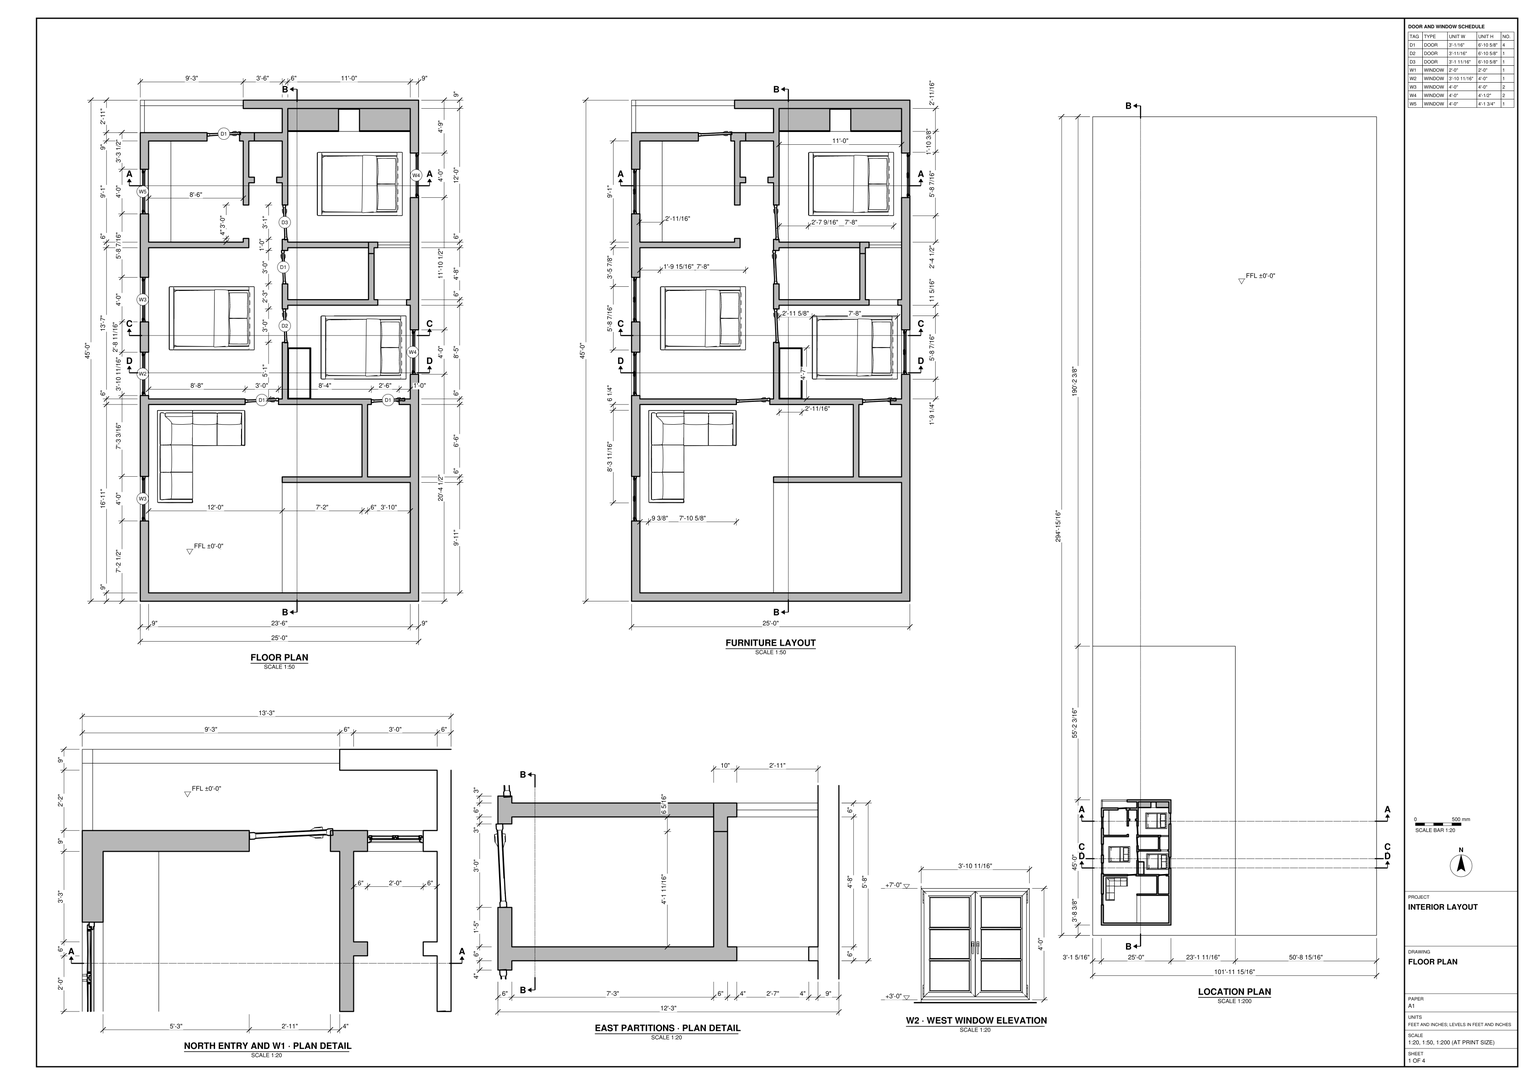
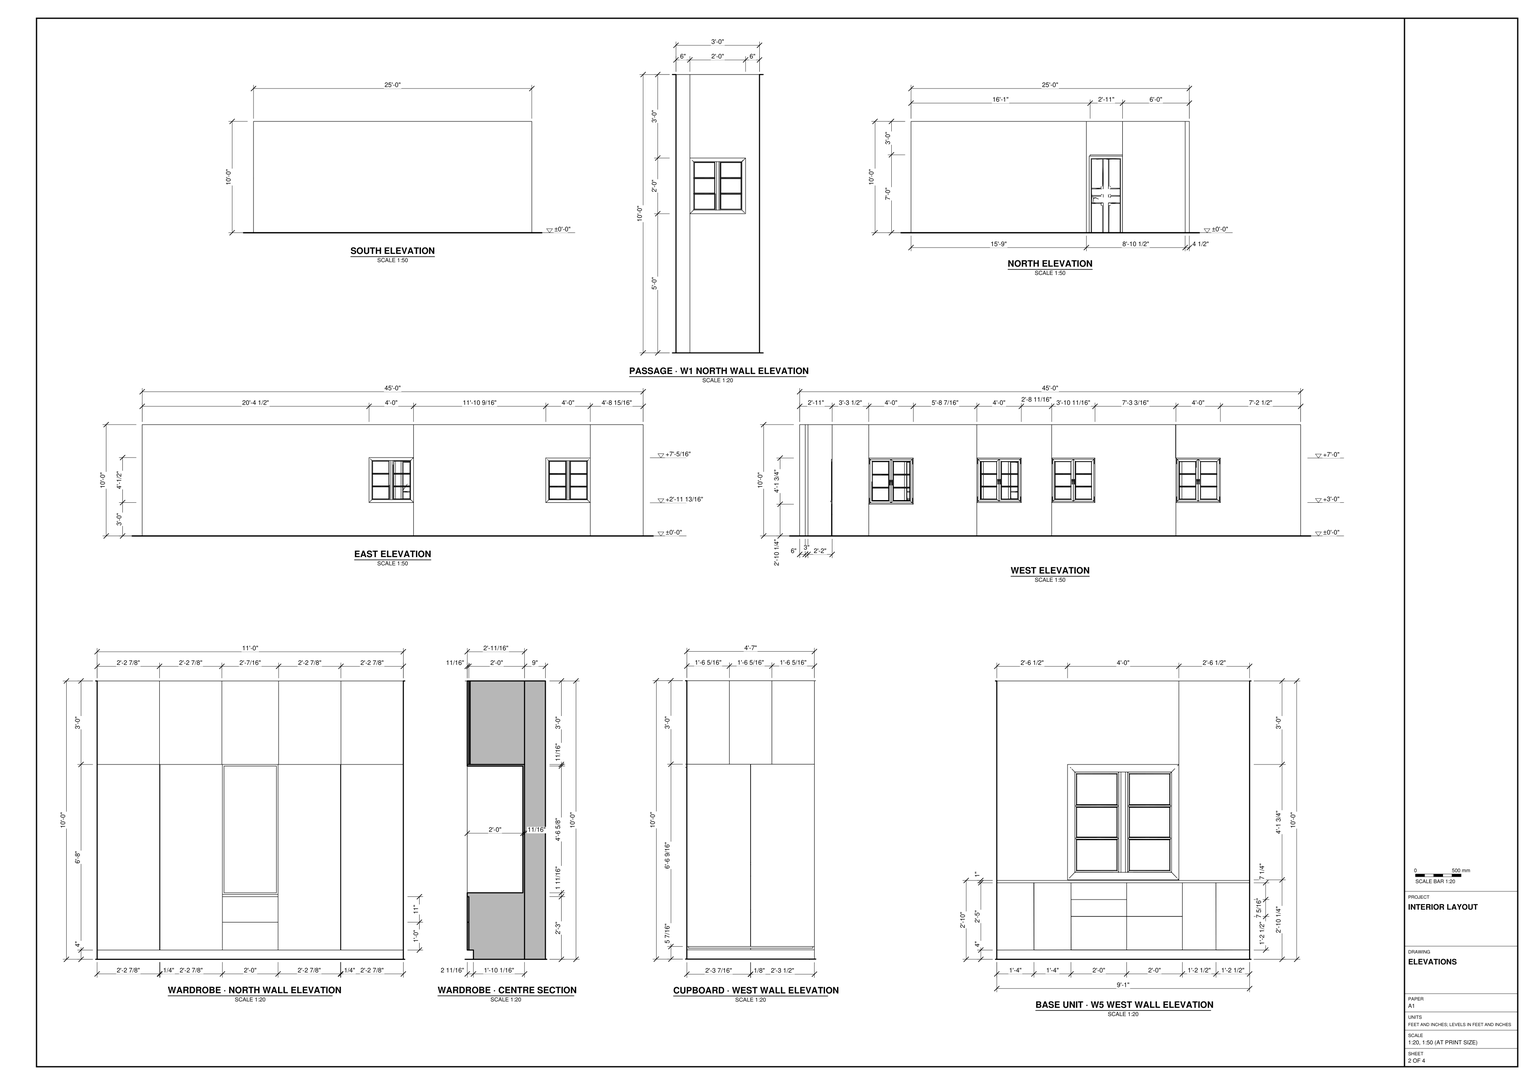
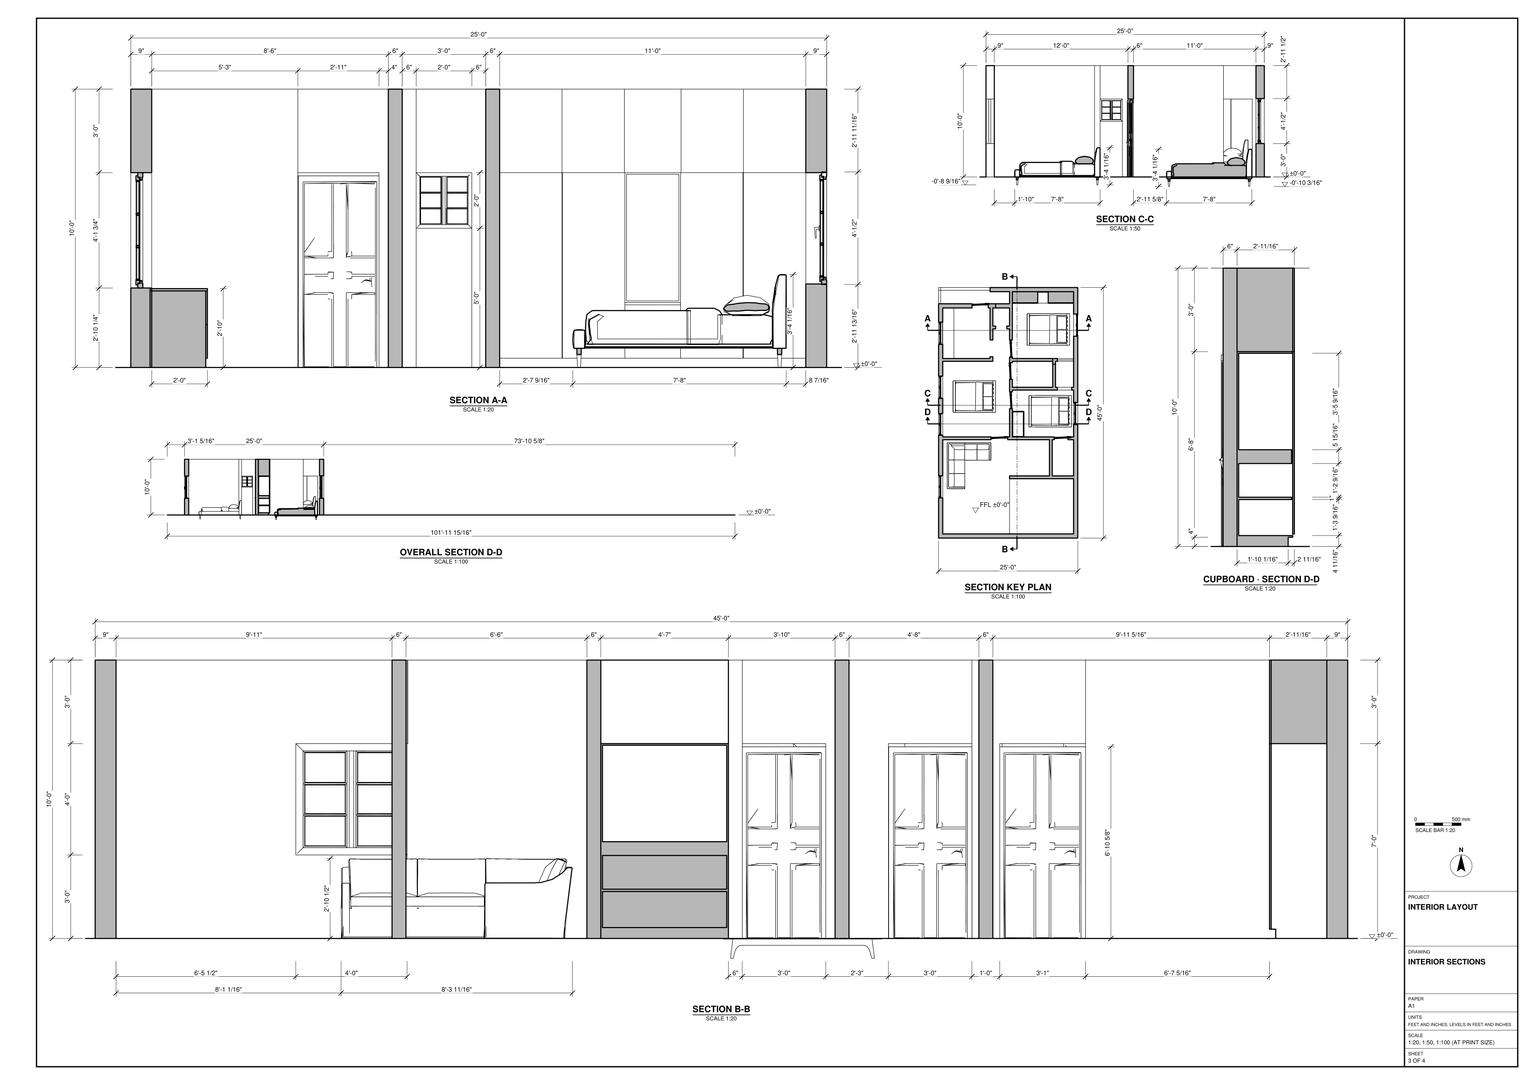
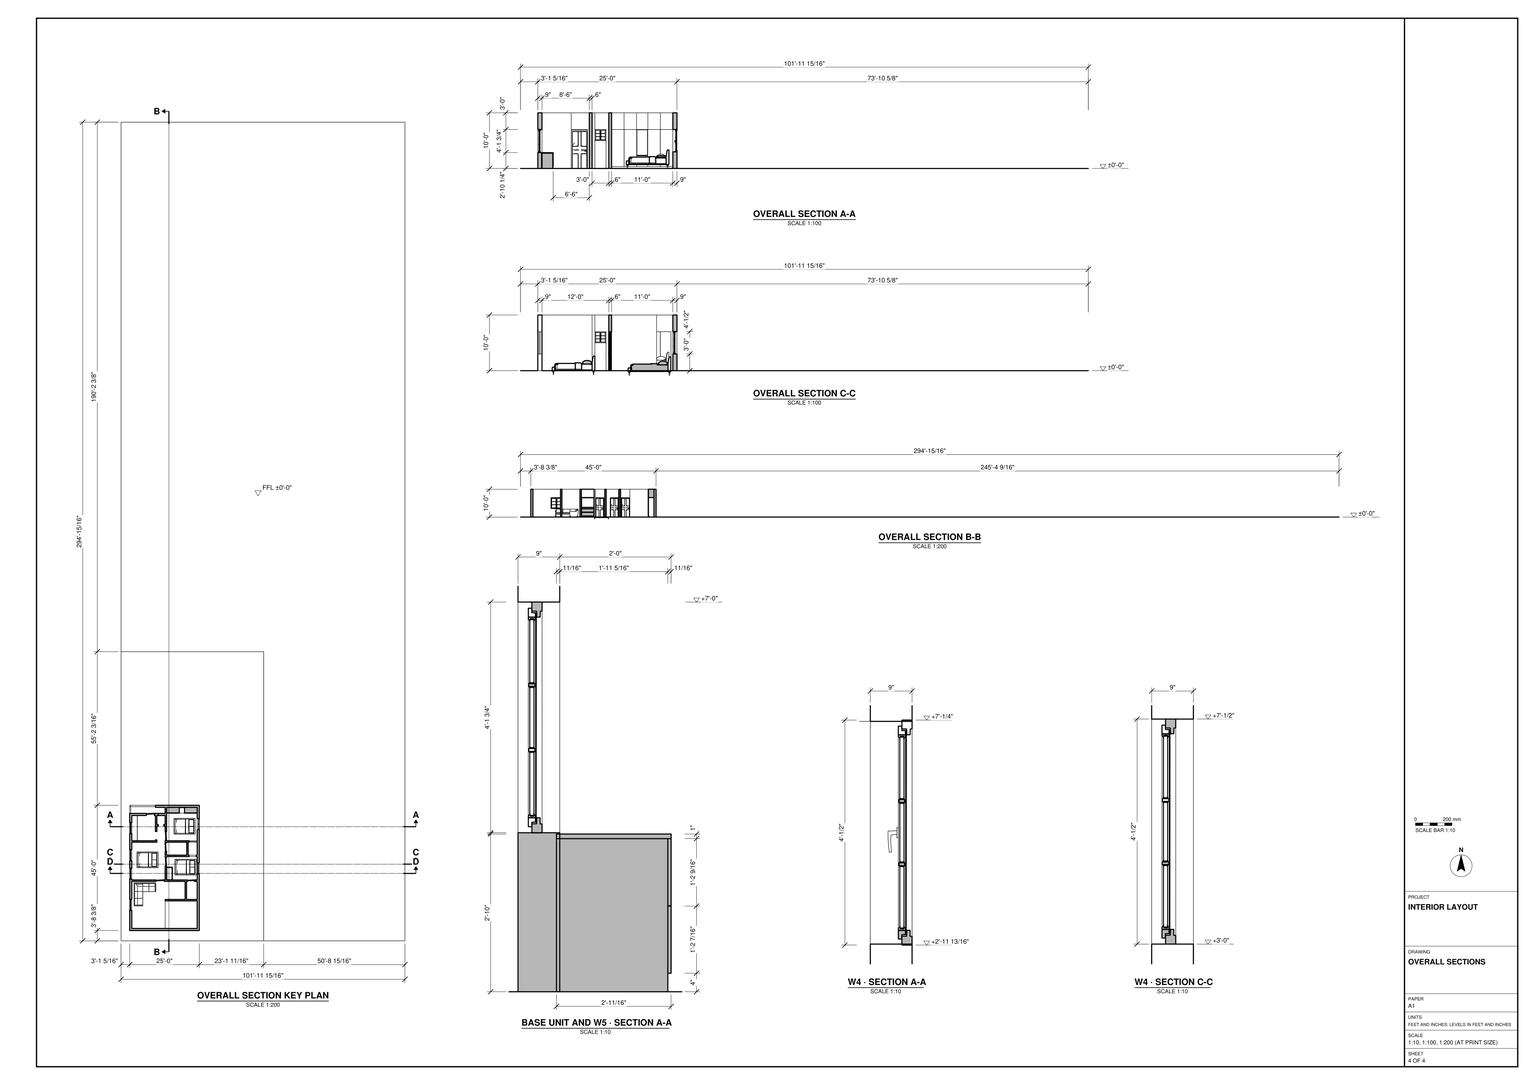
Build the furnished interior in SketchUp from task_files/diagram_01.pdf. Work in feet and inches. Use the location plan to place the 25'-0" by 45'-0" interior near the southwest corner of the ground surface. Including that surface, the overall model extents are 101'-11 15/16" along X, 294'-15/16" along Y and 10'-10 3/16" along Z. The single finished floor level is ±0'-0".

Model the floor, the stepped north entry, the perimeter walls and the internal partitions. Follow the plan for wall thicknesses, including the 9" perimeter walls and 6" partitions where indicated. Use the elevations and sections for the 10'-0" wall height, door heads and window sills. Fit the doors and framed window units into their openings, including the small high window at the north passage.

Place the three platform beds and the L-shaped sectional to match the furniture layout. Build the full-height wardrobe across the north end of the northeast bedroom, the tall cupboard against the west wall of the other east bedroom, and the low base unit beneath the northwest room's west window. Use the joinery elevations and sections for the cabinet fronts, recesses and shelf divisions.

Keep shell elements and each furniture or joinery piece in separate groups or components, and use components for repeated parts. Decor and loose items may be any suitable library components. Save one SketchUp model as output_files/single_storey_furnished_interior_with_built_in_joinery.skp.

# SketchUp Ruby script. Lengths in inches.
U = 1.inch
M = Sketchup.active_model
def pt(a) = Geom::Point3d.new(a.map { |v| v * U })
def face(e, loops, mat)
  f = e.add_face(loops[0].map { |a| pt(a) })
  loops[1..].each { |l| e.add_face(l.map { |a| pt(a) }).erase! }
  f.material = f.back_material = mat if mat
  f
end
# faces: each face lists its corners as indices into pts; further lists are holes
def faces(e, pts, list, mat = nil) = list.each { |f| face(e, (f[0].is_a?(Array) ? f : [f]).map { |l| l.map { |i| pts[i] } }, mat) }
# xy, xz, yz: faces in a plane at the given z, y or x. An outline is a flat list of corners, or four numbers for a rectangle; further outlines are holes
def ring(l) = l.size == 4 ? [[l[0], l[1]], [l[2], l[1]], [l[2], l[3]], [l[0], l[3]]] : l.each_slice(2).to_a
def flat(e, list, mat, &to3) = list.each { |f| face(e, (f[0].is_a?(Array) ? f : [f]).map { |l| ring(l).map { |u, v| to3.(u, v) } }, mat) }
def xy(e, z, list, mat = nil) = flat(e, list, mat) { |x, y| [x, y, z] }
def xz(e, y, list, mat = nil) = flat(e, list, mat) { |x, z| [x, y, z] }
def yz(e, x, list, mat = nil) = flat(e, list, mat) { |y, z| [x, y, z] }
def lines(e, pts, list) = list.each { |a, b| e.add_line(pt(pts[a]), pt(pts[b])) }
# prism: a flat outline (further loops are holes) pulled along v
def prism(e, loops, v, mat = nil)
  f = face(e, loops, mat); d = Geom::Vector3d.new(v.map { |x| x * U })
  f.pushpull(f.normal.samedirection?(d) ? d.length : -d.length)
end
def box(e, o, s, mat = nil) = prism(e, [[o, [o[0] + s[0], o[1], o[2]], [o[0] + s[0], o[1] + s[1], o[2]], [o[0], o[1] + s[1], o[2]]]], [0, 0, s[2]], mat)
def at(x, y, z, deg = 0) = Geom::Transformation.translation(pt([x, y, z])) * Geom::Transformation.rotation(ORIGIN, Z_AXIS, deg.degrees)
def axes(o, x, y, z) = Geom::Transformation.new([*x, 0, *y, 0, *z, 0, *pt(o).to_a, 1])
def part(name) = M.definitions.add(name)
# library, detail: a bought-in or finely detailed component or shape, given as its bounding box
def library(name, o, s) = part(name).tap { |d| box(d.entities, o, s) }
def detail(e, o, s) = box(e.add_group.entities, o, s)
def put(e, d, t, mat = nil) = e.add_instance(d, t).tap { |i| i.material = mat if mat }
def group(e, t, mat = nil) = e.add_group.tap { |g| g.transformation = t; g.material = mat if mat }.entities
root = M.entities
M.materials.add("[Carrera Marble]").color = [207, 207, 207]
M.materials.add("[Color M00]").color = [255, 255, 255]
M.materials.add("[Wood Lumber ButtJoined]").color = [164, 152, 112]
c1 = library("Tyler Platform Bed",[-34.22,-45.98,0],[68.44,91.98,40.05])
c2 = library("Door 243 055",[-21.32,-2.38,0],[42.64,4.76,82.63])
c3 = library("Window 46-30",[-29.96,-2.6,0],[59.92,5.19,59.84])
c4 = library("Vera Skirted Sectional",[-60.05,-44.72,0.01],[94.64,99.72,34.49])
c5 = part("Group\#16")
box(c5.entities,[0,0,0],[26.89,0.71,80])
c6 = part("Group\#15")
box(c6.entities,[0,0,0],[26.89,0.71,36])
c7 = part("Group\#17")
box(c7.entities,[0,0,0],[0.71,18.33,36],"[Color M00]")
c8 = part("Group\#24")
prism(c8.entities,[[[0.709,0,0],[0.709,14.5,0.028],[0.709,14.443,28.997],[0.709,14.443,29],[0.709,0,29]]],[-0.709,0,0],"[Color M00]")
c9 = part("Group\#22")
prism(c9.entities,[[[0.71,0,0],[0.71,16,0.03],[0.71,15.94,29],[0.71,0,29]]],[-0.71,0,0],"[Color M00]")
c10 = part("Group\#26")
box(c10.entities,[0,0,0],[0.71,24,14.47],"[Color M00]")
c11 = part("Group\#25")
box(c11.entities,[0,0,0],[0.71,24,7.23],"[Color M00]")
xy(root,0,[[615.02,0,1223.9375,0,1223.9375,3528.9375,0,3528.9375,0,1246.59,615.02,1246.59],[[0,0,615.02,1246.59],[37.3125,44.375,337.3125,584.375]],[37.3125,130.875,46.3125,178.875],[37.3125,266.07,46.3125,312.75],[328.3125,288.875,337.3125,336.875],
  [37.3125,393.4375,46.3125,393.4375,46.3125,425.375,154.3125,425.375,154.3125,435.375,148.3125,435.375,148.3125,431.375,46.3125,431.375,46.3125,461.875,37.3125,461.875],[283.3125,397.375,286.3125,419.08],[286.3125,397.375,289.3125,419.08],[37.3125,461.875,46.3125,509.875],[190.3125,471.375,196.3125,471.375,196.3125,575.375,328.3125,575.375,328.3125,527.375,337.3125,527.375,337.3125,584.375,148.3125,584.375,148.3125,575.375,190.3125,575.375,190.3125,549.375,184.3125,549.375,184.3125,540.375,190.3125,540.375,190.3125,501.375,184.3125,501.375,184.3125,495.375,190.3125,495.375],
  [328.3125,479.375,337.3125,527.375],[37.3125,509.875,46.3125,509.875,46.3125,540.375,109.3125,540.375,109.3125,549.375,37.3125,549.375],[160.3125,540.375,184.3125,544.875],[160.3125,544.875,184.3125,549.375],[37.3125,549.375,41.8125,578.375],
  [37.3125,578.375,41.8125,584.375],[41.8125,578.375,148.3125,584.375]])
xy(root,0,[[46.3125,53.375,190.3125,53.375,190.3125,178.375,276.3125,178.375,276.3125,256.375,186.3125,256.375,186.3125,262.375,190.3125,262.375,190.3125,323.375,196.3125,323.375,196.3125,317.375,220.3125,317.375,220.3125,262.375,286.3125,262.375,286.3125,256.375,282.3125,256.375,282.3125,178.375,328.3125,178.375,328.3125,256.375,316.3125,256.375,316.3125,262.375,328.3125,262.375,328.3125,363.375,196.3125,363.375,196.3125,359.375,190.3125,359.375,190.3125,386.375,196.3125,386.375,196.3125,369.375,283.3125,369.375,283.3125,425.375,196.3125,425.375,196.3125,422.375,190.3125,422.375,190.3125,434.375,196.3125,434.375,196.3125,431.375,328.3125,431.375,328.3125,551.375,196.3125,551.375,196.3125,471.375,190.3125,471.375,190.3125,495.375,184.3125,495.375,184.3125,501.375,190.3125,501.375,190.3125,540.375,154.3125,540.375,154.3125,501.375,160.3125,501.375,160.3125,495.375,154.3125,495.375,154.3125,471.375,148.3125,471.375,148.3125,540.375,144.3125,540.375,144.3125,549.375,190.3125,549.375,190.3125,575.375,148.3125,575.375,148.3125,578.375,41.8125,578.375,41.8125,549.375,109.3125,549.375,109.3125,540.375,70.3125,540.375,70.3125,431.375,148.3125,431.375,148.3125,435.375,154.3125,435.375,154.3125,425.375,46.3125,425.375,46.3125,262.375,150.3125,262.375,150.3125,256.375,46.3125,256.375],[190.3125,53.375,328.3125,172.375],[293.3125,363.375,328.3125,369.375],[289.3125,369.375,328.3125,425.375],[293.3125,425.375,328.3125,428.375],
  [293.3125,428.375,328.3125,431.375],[46.3125,431.375,70.3125,540.375],[196.3125,551.375,328.3125,575.375]],"[Carrera Marble]")
xy(root,0,[[196.3125,262.375,220.3125,317.375]],"[Color M00]")
xy(root,36,[[37.3125,345.4375,46.3125,393.4375]])
xy(root,84,[[37.3125,345.4375,46.3125,393.4375]])
xy(root,120,[[37.3125,312.75,46.3125,393.4375],[283.3125,419.08,289.3125,419.08,289.3125,425.375,293.3125,425.375,293.3125,431.375,283.3125,431.375]])
xz(root,312.75,[[37.3125,0,46.3125,120]])
xz(root,345.4375,[[37.3125,36,46.3125,84]])
xz(root,393.4375,[[37.3125,0,46.3125,36],[37.3125,84,46.3125,120]])
xz(root,419.08,[[283.3125,0,286.3125,120],[286.3125,0,289.3125,120]])
xz(root,425.375,[[289.3125,0,293.3125,120]])
xz(root,431.375,[[283.3125,0,293.3125,120]])
yz(root,37.3125,[[312.75,0,312.75,120,393.4375,120,393.4375,84,345.4375,84,345.4375,36,393.4375,36,393.4375,0]])
yz(root,46.3125,[[312.75,0,393.4375,0,393.4375,36,345.4375,36,345.4375,84,393.4375,84,393.4375,120,312.75,120]])
yz(root,283.3125,[[419.08,0,425.375,120],[425.375,0,431.375,120]])
yz(root,289.3125,[[419.08,0,425.375,120]])
yz(root,293.3125,[[425.375,0,428.375,120],[428.375,0,431.375,120]])
put(root,c1,at(273.86,494.08,0,-90))
put(root,c2,axes([193.42,341.22,0],[0.0419,-0.85678,0],[0.99881,0.04885,0],[0,0,1]))
put(root,c2,axes([191.8125,404.39,0],[0.04123,-0.84294,0],[0.99881,0.04885,0],[0,0,1]))
put(root,c2,axes([193.39,452.71,0],[0.04305,-0.88018,0],[0.99881,0.04885,0],[0,0,1]))
put(root,c2,axes([168.39,260.875,0],[-0.84224,-0.04119,0],[0.04885,-0.99881,0],[0,0,1]))
put(root,c2,axes([304.39,260.875,0],[-0.84224,-0.04119,0],[0.04885,-0.99881,0],[0,0,1]))
put(root,c2,axes([127.39,547.875,0],[-0.84224,-0.04119,0],[0.04885,-0.99881,0],[0,0,1]))
put(root,c3,axes([39.91,154.875,36],[0,-0.8011,0],[1,0,0],[0,0,0.80216]))
put(root,c3,axes([39.91,289.41,36],[0,-0.77904,0],[1,0,0],[0,0,0.80216]))
put(root,c3,axes([39.91,369.4375,36],[0,-0.8011,0],[1,0,0],[0,0,0.80216]))
put(root,c3,axes([39.91,485.875,34.24],[0,-0.8011,0],[1,0,0],[0,0,0.83154]))
put(root,c3,axes([330.91,312.875,36],[0,-0.8011,0],[1,0,0],[0,0,0.81051]))
put(root,c3,axes([172.3125,546.78,60],[-0.40055,0,0],[0,-1,0],[0,0,0.40108]))
put(root,c3,axes([334.72,503.41,35.79],[0,-0.8011,0],[1,0,0],[0,0,0.81051]))
put(root,c1,at(277.89,317.83,-10.19,-90))
put(root,c4,at(115.72,195.13,-0.01))
put(root,c1,at(114.25,349.31,-8.53,-90))
g1 = group(root,at(328.3125,336.875,0))
xy(g1,0,[[0,0,0,26.5,-4,26.5,-4,32.5,0,32.5,0,190.5,9,190.5,9,0]])
xy(g1,36,[[0,142.5,9,190.5]])
xy(g1,84,[[-35,26.5,-4,32.5],[0,142.5,9,190.5]])
xy(g1,120,[[0,0,9,0,9,190.5,0,190.5,0,32.5,-35,32.5,-35,26.5,0,26.5]])
xz(g1,0,[[0,0,9,120]])
xz(g1,26.5,[[-4,0,0,0,0,120,-35,120,-35,84,-4,84]])
xz(g1,32.5,[[-4,0,-4,84,-35,84,-35,120,0,120,0,0]])
xz(g1,142.5,[[0,36,9,84]])
xz(g1,190.5,[[0,0,9,36],[0,84,9,120]])
yz(g1,-35,[[26.5,84,32.5,120]])
yz(g1,-4,[[26.5,0,32.5,84]])
yz(g1,0,[[0,0,26.5,120],[32.5,0,88.5,120],[88.5,0,91.5,120],[91.5,0,94.5,120],[94.5,0,94.5,120,190.5,120,190.5,84,142.5,84,142.5,36,190.5,36,190.5,0]])
yz(g1,9,[[0,0,190.5,0,190.5,36,142.5,36,142.5,84,190.5,84,190.5,120,0,120]])
g2 = group(root,at(190.3125,359.375,0))
xy(g2,0,[[0,0,0,27,6,27,6,10,93,10,93,59.71,99,59.71,99,10,103,10,103,4,6,4,6,0]])
xy(g2,72,[[93,38,99,59.71]])
xy(g2,84,[[0,-36,6,0],[0,27,6,63]])
xy(g2,96,[[93,38,99,59.71]])
xy(g2,120,[[0,-36,6,-36,6,4,103,4,103,10,99,10,99,59.71,93,59.71,93,10,6,10,6,63,0,63]])
xz(g2,-36,[[0,84,6,120]])
xz(g2,0,[[0,0,6,84]])
xz(g2,4,[[6,0,103,120]])
xz(g2,10,[[6,0,93,120],[99,0,103,120]])
xz(g2,27,[[0,0,6,84]])
xz(g2,38,[[93,72,99,96]])
xz(g2,59.71,[[93,0,99,72],[93,96,99,120]])
xz(g2,63,[[0,84,6,120]])
yz(g2,0,[[0,0,0,84,-36,84,-36,120,63,120,63,84,27,84,27,0]])
yz(g2,6,[[0,0,4,0,4,120,-36,120,-36,84,0,84],[10,0,27,0,27,84,63,84,63,120,10,120]])
yz(g2,93,[[10,0,10,120,59.71,120,59.71,96,38,96,38,72,59.71,72,59.71,0]])
yz(g2,99,[[10,0,59.71,0,59.71,72,38,72,38,96,59.71,96,59.71,120,10,120]])
yz(g2,103,[[4,0,10,120]])
g3 = group(root,at(190.3125,422.375,0))
xy(g3,0,[[0,0,0,12,6,12,6,9,93,9,93,3,6,3,6,0]])
xy(g3,84,[[0,12,6,49]])
xy(g3,120,[[0,0,6,0,6,3,93,3,93,9,6,9,6,49,0,49]])
xz(g3,0,[[0,0,6,120]])
xz(g3,3,[[6,0,93,120]])
xz(g3,9,[[6,0,93,120]])
xz(g3,12,[[0,0,6,84]])
xz(g3,49,[[0,84,6,120]])
yz(g3,0,[[0,0,0,120,49,120,49,84,12,84,12,0]])
yz(g3,6,[[0,0,3,120],[9,0,12,0,12,84,49,84,49,120,9,120]])
yz(g3,93,[[3,0,9,120]])
g4 = group(root,at(37.3125,393.4375,0))
xy(g4,0,[[0,0,0,116.4375,9,116.4375,9,37.9375,111,37.9375,111,41.9375,117,41.9375,117,31.9375,9,31.9375,9,0]])
xy(g4,34.27,[[0,68.4375,9,116.4375]])
xy(g4,84,[[111,41.9375,117,77.9375],[0,68.4375,9,116.4375]])
xy(g4,120,[[0,0,9,0,9,31.9375,117,31.9375,117,77.9375,111,77.9375,111,37.9375,9,37.9375,9,116.4375,0,116.4375]])
xz(g4,0,[[0,0,9,120]])
xz(g4,31.9375,[[9,0,117,120]])
xz(g4,37.9375,[[9,0,111,120]])
xz(g4,41.9375,[[111,0,117,84]])
xz(g4,68.4375,[[0,34.27,9,84]])
xz(g4,77.9375,[[111,84,117,120]])
xz(g4,116.4375,[[0,0,9,34.27],[0,84,9,120]])
yz(g4,0,[[0,0,0,120,116.4375,120,116.4375,84,68.4375,84,68.4375,34.27,116.4375,34.27,116.4375,0]])
yz(g4,9,[[0,0,31.9375,120],[37.9375,0,116.4375,0,116.4375,34.27,68.4375,34.27,68.4375,84,116.4375,84,116.4375,120,37.9375,120]])
yz(g4,111,[[37.9375,0,37.9375,120,77.9375,120,77.9375,84,41.9375,84,41.9375,0]])
yz(g4,117,[[31.9375,0,41.9375,0,41.9375,84,77.9375,84,77.9375,120,31.9375,120]])
g5 = group(root,at(37.3125,509.875,0))
prism(g5,[[[4.5,39.5,0],[72,39.5,0],[72,30.5,0],[9,30.5,0],[9,0,0],[0,0,0],[0,39.5,0]]],[0,0,120])
g6 = group(root,at(144.3125,471.375,0))
xy(g6,0,[[4,0,4,69,0,69,0,78,16,78,16,69,10,69,10,30,16,30,16,24,10,24,10,0]])
xy(g6,84,[[-35,69,0,78]])
xy(g6,120,[[4,0,10,0,10,24,16,24,16,30,10,30,10,69,16,69,16,78,-35,78,-35,69,4,69]])
xz(g6,0,[[4,0,10,120]])
xz(g6,24,[[10,0,16,120]])
xz(g6,30,[[10,0,16,120]])
xz(g6,69,[[0,0,4,0,4,120,-35,120,-35,84,0,84],[10,0,16,120]])
xz(g6,78,[[0,0,0,84,-35,84,-35,120,16,120,16,0]])
yz(g6,-35,[[69,84,78,120]])
yz(g6,0,[[69,0,78,84]])
yz(g6,4,[[0,0,69,120]])
yz(g6,10,[[0,0,24,120],[30,0,69,120]])
yz(g6,16,[[24,0,30,120],[69,0,73.5,120],[73.5,0,78,120]])
g7 = group(root,at(37.3125,178.875,0))
xy(g7,0,[[0,0,0,133.875,9,133.875,9,83.5,113,83.5,113,77.5,9,77.5,9,0]])
xy(g7,36,[[0,87.2,9,133.875]])
xy(g7,84,[[0,87.2,9,133.875]])
xy(g7,120,[[0,0,9,0,9,77.5,113,77.5,113,83.5,9,83.5,9,133.875,0,133.875]])
xz(g7,0,[[0,0,9,120]])
xz(g7,77.5,[[9,0,113,120]])
xz(g7,83.5,[[9,0,113,120]])
xz(g7,87.2,[[0,36,9,84]])
xz(g7,133.875,[[0,0,9,36],[0,84,9,120]])
yz(g7,0,[[0,0,0,120,133.875,120,133.875,84,87.2,84,87.2,36,133.875,36,133.875,0]])
yz(g7,9,[[0,0,77.5,120],[83.5,0,133.875,0,133.875,36,87.2,36,87.2,84,133.875,84,133.875,120,83.5,120]])
yz(g7,113,[[77.5,0,83.5,120]])
g8 = group(root,at(37.3125,44.375,0))
xy(g8,0,[[0,0,0,134.5,9,134.5,9,9,291,9,291,128,153,128,153,134,239,134,239,212,149,212,149,218,153,218,153,279,159,279,159,218,249,218,249,212,245,212,245,134,291,134,291,212,279,212,279,218,291,218,291,292.5,300,292.5,300,0]])
xy(g8,36,[[0,86.5,9,134.5],[291,244.5,300,292.5]])
xy(g8,84,[[0,86.5,9,134.8125],[113,212,149,218],[249,212,279,218]])
xy(g8,84.5,[[291,244.5,300,292.5]])
xy(g8,120,[[[0,0,300,0,300,292.5,291,292.5,291,218,159,218,159,279,153,279,153,218,113,218,113,212,239,212,239,134,153,134,153,128,291,128,291,9,9,9,9,134.8125,0,134.8125],[245,134,291,212]]])
xz(g8,0,[[0,0,300,120]])
xz(g8,9,[[9,0,153,120],[153,0,291,120]])
xz(g8,86.5,[[0,36,9,84]])
xz(g8,128,[[153,0,291,120]])
xz(g8,134,[[153,0,239,120],[245,0,291,120]])
xz(g8,134.5,[[0,0,9,36]])
xz(g8,134.8125,[[0,84,9,120]])
xz(g8,212,[[149,0,239,0,239,120,113,120,113,84,149,84],[245,0,249,120],[279,0,291,0,291,120,249,120,249,84,279,84]])
xz(g8,218,[[149,0,149,84,113,84,113,120,153,120,153,0],[159,0,249,120],[279,0,279,84,249,84,249,120,291,120,291,0]])
xz(g8,244.5,[[291,36,300,84.5]])
xz(g8,279,[[153,0,159,120]])
xz(g8,292.5,[[291,0,300,36],[291,84.5,300,120]])
yz(g8,0,[[0,0,0,120,134.8125,120,134.8125,84,86.5,84,86.5,36,134.5,36,134.5,0]])
yz(g8,9,[[9,0,134.5,0,134.5,36,86.5,36,86.5,84,134.8125,84,134.8125,120,9,120]])
yz(g8,113,[[212,84,218,120]])
yz(g8,149,[[212,0,218,84]])
yz(g8,153,[[128,0,134,120],[218,0,279,120]])
yz(g8,159,[[218,0,279,120]])
yz(g8,239,[[134,0,212,120]])
yz(g8,245,[[134,0,212,120]])
yz(g8,249,[[212,0,218,84]])
yz(g8,279,[[212,0,218,84]])
yz(g8,291,[[9,0,128,120],[134,0,212,120],[218,0,218,120,292.5,120,292.5,84.5,244.5,84.5,244.5,36,292.5,36,292.5,0]])
yz(g8,300,[[0,0,292.5,0,292.5,36,244.5,36,244.5,84.5,292.5,84.5,292.5,120,0,120]])
g9 = group(root,at(148.3125,471.375,0))
xy(g9,0,[[42,0,42,24,36,24,36,30,42,30,42,69,12,69,12,78,42,78,42,104,0,104,0,113,189,113,189,56,180,56,180,104,48,104,48,0]])
xy(g9,60,[[12,69,36,78]])
xy(g9,84,[[12,24,36,30],[12,69,36,78]])
xy(g9,120,[[42,0,48,0,48,104,180,104,180,56,189,56,189,113,0,113,0,104,42,104,42,78,12,78,12,69,42,69,42,30,12,30,12,24,42,24]])
xz(g9,0,[[42,0,48,120]])
xz(g9,24,[[36,0,42,0,42,120,12,120,12,84,36,84]])
xz(g9,30,[[36,0,36,84,12,84,12,120,42,120,42,0]])
xz(g9,56,[[180,0,189,120]])
xz(g9,69,[[12,0,42,0,42,120,12,120,12,84,36,84,36,60,12,60]])
xz(g9,78,[[12,0,12,60,36,60,36,84,12,84,12,120,42,120,42,0]])
xz(g9,104,[[0,0,42,120],[48,0,180,120]])
xz(g9,113,[[0,0,189,120]])
yz(g9,0,[[104,0,107,120],[107,0,113,120]])
yz(g9,12,[[69,0,78,60],[24,84,30,120],[69,84,78,120]])
yz(g9,36,[[24,0,30,84],[69,60,78,84]])
yz(g9,42,[[0,0,24,120],[30,0,69,120],[78,0,104,120]])
yz(g9,48,[[0,0,104,120]])
yz(g9,180,[[56,0,104,120]])
yz(g9,189,[[56,0,113,120]])
g10 = group(root,at(196.3125,551.375,0))
xy(g10,0,[[0,1.97,132,24]])
xy(g10,4,[[0,0,132,1.97]])
xy(g10,27,[[54,-0.71,78,0]],"[Wood Lumber ButtJoined]")
xy(g10,28.68,[[54.71,-0.71,77.29,23.29]],"[Wood Lumber ButtJoined]")
xy(g10,83.29,[[54.71,-0.71,77.29,23.29]],"[Wood Lumber ButtJoined]")
xy(g10,84,[[54,-0.71,78,-0.71,78,0,132,0,132,24,0,24,0,0,54,0]])
xz(g10,-0.71,[[54,27,78,27.97],[[54,27.97,78,84],[54.71,28.68,77.29,83.29]]],"[Wood Lumber ButtJoined]")
xz(g10,0,[[0,4,28.81,84],[28.81,4,54,84],[54,4,78,15.99],[78,4,105.11,84],[105.11,4,132,84],
  [54,15.99,78,27]])
xz(g10,1.97,[[0,0,132,4]],"[Wood Lumber ButtJoined]")
xz(g10,23.29,[[54.71,28.68,77.29,83.29]],"[Wood Lumber ButtJoined]")
xz(g10,24,[[0,0,132,84]])
yz(g10,0,[[1.97,0,1.97,4,0,4,0,84,24,84,24,0]])
yz(g10,54,[[-0.71,27.97,0,84]])
yz(g10,54,[[-0.71,27,0,27.97]],"[Wood Lumber ButtJoined]")
yz(g10,54.71,[[-0.71,28.68,23.29,83.29]],"[Wood Lumber ButtJoined]")
yz(g10,77.29,[[-0.71,28.68,23.29,83.29]],"[Wood Lumber ButtJoined]")
yz(g10,78,[[-0.71,27.97,0,84]])
yz(g10,78,[[-0.71,27,0,27.97]],"[Wood Lumber ButtJoined]")
yz(g10,132,[[1.97,0,24,0,24,84,0,84,0,4,1.97,4]])
g11 = group(g10,at(105.11,-0.71,4),"[Wood Lumber ButtJoined]")
box(g11,[0,0,0],[26.89,0.71,80])
put(g10,c5,at(78,-0.71,4),"[Wood Lumber ButtJoined]")
put(g10,c5,at(0,-0.71,4),"[Wood Lumber ButtJoined]")
put(g10,c5,at(27.11,-0.71,4),"[Wood Lumber ButtJoined]")
g12 = group(g10,at(54,-0.71,4),"[Wood Lumber ButtJoined]")
box(g12,[0,0,0],[24,0.71,11.99])
g13 = group(g10,at(54,-0.71,15.99),"[Wood Lumber ButtJoined]")
box(g13,[0,0,0],[24,0.71,11.01])
put(g10,c6,at(0,-0.71,84),"[Wood Lumber ButtJoined]")
put(g10,c6,at(26.89,-0.71,84),"[Wood Lumber ButtJoined]")
put(g10,c6,at(105.11,-0.71,84),"[Wood Lumber ButtJoined]")
put(g10,c6,at(78.22,-0.71,84),"[Wood Lumber ButtJoined]")
put(g10,c6,axes([53.78,-0.71,84],[0.90934,0,0],[0,1.77,0],[0,0,1]),"[Wood Lumber ButtJoined]")
g14 = group(root,at(196.3125,551.375,84))
box(g14,[0,0,0],[132,24,36],"[Wood Lumber ButtJoined]")
g15 = group(root,at(221.02,317.375,0,180))
xy(g15,0,[[2.68,0,24.71,55]],"[Color M00]")
xy(g15,4,[[0.71,0,2.68,55]],"[Color M00]")
xy(g15,4.71,[[0.71,0.71,24,54.29]],"[Color M00]")
xy(g15,20.24,[[1.21,0.71,24,54.29]],"[Color M00]")
xy(g15,21.24,[[1.21,0.71,24,54.29]],"[Color M00]")
xy(g15,35.77,[[1.21,0.71,24,54.29]],"[Color M00]")
xy(g15,41.71,[[1.21,0.71,24,54.29]],"[Color M00]")
xy(g15,83.29,[[0.71,0.71,24,54.29]],"[Color M00]")
xy(g15,84,[[0.71,0,24.71,55]],"[Color M00]")
xz(g15,0,[[2.68,0,24.71,0,24.71,84,0.71,84,0.71,4,2.68,4]],"[Color M00]")
xz(g15,0.71,[[0.71,4.71,0.71,35.77,24,35.77,24,21.24,1.21,21.24,1.21,20.24,24,20.24,24,4.71],[0.71,35.77,1.21,40.71],[0.71,40.71,0.71,83.29,24,83.29,24,41.71,1.21,41.71,1.21,40.71]],"[Color M00]")
xz(g15,54.29,[[0.71,4.71,24,4.71,24,20.24,1.21,20.24,1.21,21.24,24,21.24,24,35.77,0.71,35.77],[0.71,35.77,1.21,40.71],[0.71,40.71,1.21,40.71,1.21,41.71,24,41.71,24,83.29,0.71,83.29]],"[Color M00]")
xz(g15,55,[[2.68,0,2.68,4,0.71,4,0.71,84,24.71,84,24.71,0]],"[Color M00]")
yz(g15,0.71,[[0,4,0,84,27.5,84,27.5,83.29,0.71,83.29,0.71,4.71,27.5,4.71,27.5,4],[27.5,4,27.5,4.71,54.29,4.71,54.29,83.29,27.5,83.29,27.5,84,55,84,55,4]],"[Color M00]")
yz(g15,1.21,[[0.71,20.24,54.29,21.24],[0.71,35.77,54.29,40.71],[0.71,40.71,54.29,41.71]],"[Color M00]")
yz(g15,2.68,[[0,0,55,4]],"[Color M00]")
yz(g15,24,[[0.71,4.71,54.29,20.24],[0.71,21.24,54.29,35.77],[0.71,41.71,54.29,83.29]],"[Color M00]")
yz(g15,24.71,[[0,0,55,84]],"[Color M00]")
g16 = group(g15,at(0,0,5.42))
prism(g16,[[[0,27.48,78.58],[0,27.48,0],[0,0,0],[0,0,31.0625],[0,0,36],[0,0,78.58]]],[0.71,0,0])
g17 = group(g15,at(0,28.21,5.42))
prism(g17,[[[0,26.79,78.58],[0,26.79,0],[0,-0.625,0],[0,-0.625,36],[0,-0.625,78.58]]],[0.71,0,0])
g18 = group(root,at(221.02,317.375,84,180))
xy(g18,0,[[0.71,0,24.71,55]],"[Color M00]")
xy(g18,36,[[0.71,0,24.71,55]],"[Color M00]")
xz(g18,0,[[0.71,0,24.71,36]],"[Color M00]")
xz(g18,55,[[0.71,0,24.71,36]],"[Color M00]")
yz(g18,0.71,[[0,0,18.33,36],[18.33,0,55,36]],"[Color M00]")
yz(g18,24.71,[[0,0,55,36]],"[Color M00]")
put(g18,c7,at(0,18.33,0))
put(g18,c7,at(0,36.67,0))
put(g18,c7,at(0,0,0))
put(root,c8,at(69.6,525.875,4))
put(root,c9,at(69.6,431.375,4))
put(root,c8,at(69.6,511.375,4))
g19 = group(root,at(45.6,431.375,0))
xy(g19,0,[[0,0,24,109]],"[Color M00]")
xy(g19,33,[[0,0,24,109]],"[Color M00]")
xz(g19,0,[[0,0,24,33]],"[Color M00]")
xz(g19,109,[[0,0,24,33]],"[Color M00]")
yz(g19,0,[[0,0,30.5,33],[30.5,0,78.5,33],[78.5,0,109,33]],"[Color M00]")
yz(g19,24,[[0,0,109,0,109,4.0625,32,4.0625,16,4.03,0,4],[0,4,16,4.03,15.94,33,0,33],[16,4.03,32,4.0625,32,33,15.94,33],[32,4.0625,56,18.53],[56,4.0625,80,18.53],
  [80,4.0625,94.5,33],[94.5,4.0625,109,33],[32,18.53,56,25.77],[56,18.53,80,33],[32,25.77,56,33]],"[Color M00]")
put(g19,c10,at(24,56,4))
put(g19,c10,at(24,56,18.53))
put(g19,c10,at(24,32,4))
put(g19,c11,at(24,32,18.53))
put(g19,c11,at(24,32,25.77))
g20 = group(g19,at(0,0,33))
prism(g20,[[[24.71,0,0],[0,0,0],[0,30.5,0],[0,78.5,0],[0,109,0],[24.71,109,0]]],[0,0,1],"[Color M00]")
put(root,c9,at(69.6,447.43,4))
